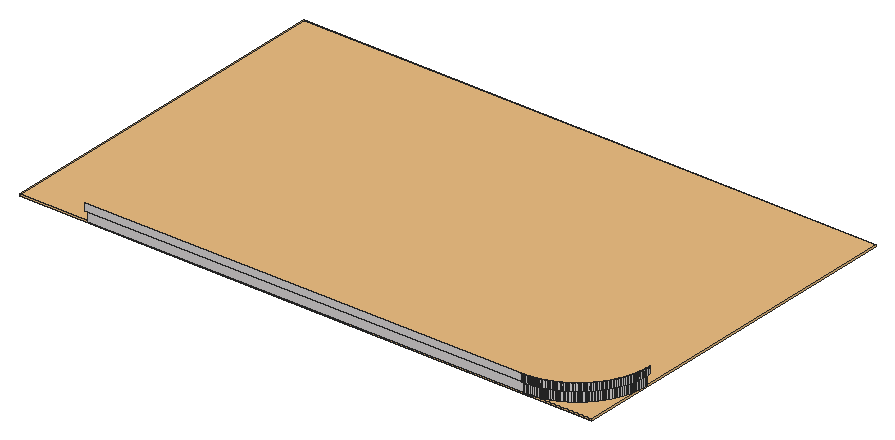
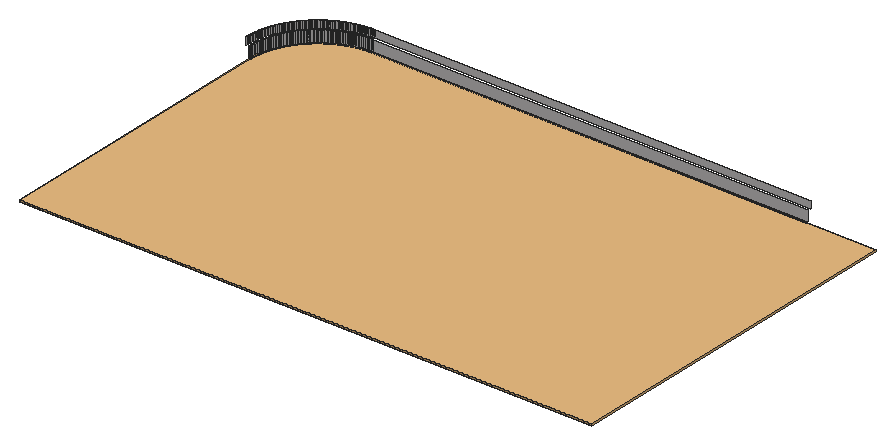
# SketchUp Ruby script. Lengths in inches.
U = 1.inch
M = Sketchup.active_model
def pt(a) = Geom::Point3d.new(a.map { |v| v * U })
def face(e, loops, mat)
  f = e.add_face(loops[0].map { |a| pt(a) })
  loops[1..].each { |l| e.add_face(l.map { |a| pt(a) }).erase! }
  f.material = f.back_material = mat if mat
  f
end
# faces: each face lists its corners as indices into pts; further lists are holes
def faces(e, pts, list, mat = nil) = list.each { |f| face(e, (f[0].is_a?(Array) ? f : [f]).map { |l| l.map { |i| pts[i] } }, mat) }
# xy, xz, yz: faces in a plane at the given z, y or x. An outline is a flat list of corners, or four numbers for a rectangle; further outlines are holes
def ring(l) = l.size == 4 ? [[l[0], l[1]], [l[2], l[1]], [l[2], l[3]], [l[0], l[3]]] : l.each_slice(2).to_a
def flat(e, list, mat, &to3) = list.each { |f| face(e, (f[0].is_a?(Array) ? f : [f]).map { |l| ring(l).map { |u, v| to3.(u, v) } }, mat) }
def xy(e, z, list, mat = nil) = flat(e, list, mat) { |x, y| [x, y, z] }
def xz(e, y, list, mat = nil) = flat(e, list, mat) { |x, z| [x, y, z] }
def yz(e, x, list, mat = nil) = flat(e, list, mat) { |y, z| [x, y, z] }
def lines(e, pts, list) = list.each { |a, b| e.add_line(pt(pts[a]), pt(pts[b])) }
# prism: a flat outline (further loops are holes) pulled along v
def prism(e, loops, v, mat = nil)
  f = face(e, loops, mat); d = Geom::Vector3d.new(v.map { |x| x * U })
  f.pushpull(f.normal.samedirection?(d) ? d.length : -d.length)
end
def box(e, o, s, mat = nil) = prism(e, [[o, [o[0] + s[0], o[1], o[2]], [o[0] + s[0], o[1] + s[1], o[2]], [o[0], o[1] + s[1], o[2]]]], [0, 0, s[2]], mat)
def at(x, y, z, deg = 0) = Geom::Transformation.translation(pt([x, y, z])) * Geom::Transformation.rotation(ORIGIN, Z_AXIS, deg.degrees)
def axes(o, x, y, z) = Geom::Transformation.new([*x, 0, *y, 0, *z, 0, *pt(o).to_a, 1])
def part(name) = M.definitions.add(name)
# library, detail: a bought-in or finely detailed component or shape, given as its bounding box
def library(name, o, s) = part(name).tap { |d| box(d.entities, o, s) }
def detail(e, o, s) = box(e.add_group.entities, o, s)
def put(e, d, t, mat = nil) = e.add_instance(d, t).tap { |i| i.material = mat if mat }
def group(e, t, mat = nil) = e.add_group.tap { |g| g.transformation = t; g.material = mat if mat }.entities
root = M.entities
M.materials.add("Outer Light - 1").color = [251, 216, 141]
M.materials.add("[Quartz Light Brown]").color = [215, 212, 212]
c1 = library("Group\#52",[-0.5,-0.5,0],[314,195,1])
xz(root,281.2,[[225,493,464,497],[464,493,464.52,497]],"[Quartz Light Brown]")
xz(root,282.7,[[225,487,464,493],[464,487,464.5,493]],"[Quartz Light Brown]")
xz(root,283.7,[[225,486,464,487],[464,486,464.48,487]],"[Quartz Light Brown]")
yz(root,501,[[320.22,486,320.7,487]],"[Quartz Light Brown]")
yz(root,502,[[320.2,487,320.7,493]],"[Quartz Light Brown]")
yz(root,503.5,[[320.18,493,320.7,497]],"[Quartz Light Brown]")
p = [[464.48,283.7,486],[464.97,283.71,486],[464.97,283.71,487],[464.48,283.7,487],[465.45,283.73,486],[465.45,283.73,487],
  [465.9375,283.75,486],[465.9375,283.75,487],[466.42,283.78,486],[466.42,283.78,487],[466.9,283.82,486],[466.9,283.82,487],
  [467.39,283.86,486],[467.39,283.86,487],[467.87,283.9,486],[467.87,283.9,487],[468.35,283.96,486],[468.35,283.96,487],
  [468.83,284.02,486],[468.83,284.02,487],[469.31,284.08,486],[469.31,284.08,487],[469.79,284.16,486],[469.79,284.16,487],
  [470.27,284.24,486],[470.27,284.24,487],[470.74,284.32,486],[470.74,284.32,487],[471.22,284.41,486],[471.22,284.41,487],
  [471.69,284.51,486],[471.69,284.51,487],[472.17,284.61,486],[472.17,284.61,487],[472.64,284.72,486],[472.64,284.72,487],
  [473.11,284.84,486],[473.11,284.84,487],[473.58,284.96,486],[473.58,284.96,487],[474.04,285.09,486],[474.04,285.09,487],
  [474.51,285.22,486],[474.51,285.22,487],[474.97,285.37,486],[474.97,285.37,487],[475.43,285.51,486],[475.43,285.51,487],
  [475.89,285.66,486],[475.89,285.66,487],[476.35,285.82,486],[476.35,285.82,487],[476.81,285.99,486],[476.81,285.99,487],
  [477.26,286.16,486],[477.26,286.16,487],[477.71,286.34,486],[477.71,286.34,487],[478.16,286.52,486],[478.16,286.52,487],
  [478.61,286.71,486],[478.61,286.71,487],[479.05,286.9,486],[479.05,286.9,487],[479.49,287.1,486],[479.49,287.1,487],
  [479.93,287.31,486],[479.93,287.31,487],[480.36,287.52,486],[480.36,287.52,487],[480.8,287.73,486],[480.8,287.73,487],
  [481.23,287.96,486],[481.23,287.96,487],[481.65,288.18,486],[481.65,288.18,487],[482.08,288.42,486],[482.08,288.42,487],
  [482.5,288.66,486],[482.5,288.66,487],[482.92,288.9,486],[482.92,288.9,487],[483.33,289.15,486],[483.33,289.15,487],
  [483.74,289.41,486],[483.74,289.41,487],[484.15,289.67,486],[484.15,289.67,487],[484.56,289.9375,486],[484.56,289.9375,487],
  [484.96,290.21,486],[484.96,290.21,487],[485.35,290.49,486],[485.35,290.49,487],[485.75,290.77,486],[485.75,290.77,487],
  [486.14,291.05,486],[486.14,291.05,487],[486.52,291.35,486],[486.52,291.35,487],[486.91,291.64,486],[486.91,291.64,487],
  [487.28,291.95,486],[487.28,291.95,487],[487.66,292.25,486],[487.66,292.25,487],[488.03,292.57,486],[488.03,292.57,487],
  [488.4,292.88,486],[488.4,292.88,487],[488.76,293.2,486],[488.76,293.2,487],[489.12,293.53,486],[489.12,293.53,487],
  [489.47,293.86,486],[489.47,293.86,487],[489.82,294.2,486],[489.82,294.2,487],[490.16,294.54,486],[490.16,294.54,487],
  [490.5,294.88,486],[490.5,294.88,487],[490.84,295.23,486],[490.84,295.23,487],[491.17,295.59,486],[491.17,295.59,487],
  [491.5,295.94,486],[491.5,295.94,487],[491.82,296.31,486],[491.82,296.31,487],[492.14,296.67,486],[492.14,296.67,487],
  [492.45,297.04,486],[492.45,297.04,487],[492.75,297.42,486],[492.75,297.42,487],[493.06,297.79,486],[493.06,297.79,487],
  [493.35,298.18,486],[493.35,298.18,487],[493.65,298.5625,486],[493.65,298.5625,487],[493.93,298.95,486],[493.93,298.95,487],
  [494.22,299.35,486],[494.22,299.35,487],[494.49,299.74,486],[494.49,299.74,487],[494.76,300.14,486],[494.76,300.14,487],
  [495.03,300.55,486],[495.03,300.55,487],[495.29,300.96,486],[495.29,300.96,487],[495.55,301.37,486],[495.55,301.37,487],
  [495.8,301.78,486],[495.8,301.78,487],[496.04,302.2,486],[496.04,302.2,487],[496.28,302.62,486],[496.28,302.62,487],
  [496.52,303.05,486],[496.52,303.05,487],[496.74,303.47,486],[496.74,303.47,487],[496.97,303.9,486],[496.97,303.9,487],
  [497.18,304.34,486],[497.18,304.34,487],[497.4,304.77,486],[497.4,304.77,487],[497.6,305.21,486],[497.6,305.21,487],
  [497.8,305.65,486],[497.8,305.65,487],[498,306.1,486],[498,306.1,487],[498.18,306.54,486],[498.18,306.54,487],
  [498.37,306.99,486],[498.37,306.99,487],[498.54,307.44,486],[498.54,307.44,487],[498.71,307.89,486],[498.71,307.89,487],
  [498.88,308.35,486],[498.88,308.35,487],[499.04,308.81,486],[499.04,308.81,487],[499.1875,309.27,486],[499.1875,309.27,487],
  [499.34,309.73,486],[499.34,309.73,487],[499.48,310.19,486],[499.48,310.19,487],[499.61,310.66,486],[499.61,310.66,487],
  [499.74,311.125,486],[499.74,311.125,487],[499.86,311.59,486],[499.86,311.59,487],[499.98,312.0625,486],[499.98,312.0625,487],
  [500.09,312.54,486],[500.09,312.54,487],[500.19,313.01,486],[500.19,313.01,487],[500.29,313.48,486],[500.29,313.48,487],
  [500.38,313.96,486],[500.38,313.96,487],[500.47,314.44,486],[500.47,314.44,487],[500.54,314.91,486],[500.54,314.91,487],
  [500.62,315.39,486],[500.62,315.39,487],[500.68,315.87,486],[500.68,315.87,487],[500.74,316.35,486],[500.74,316.35,487],
  [500.8,316.83,486],[500.8,316.83,487],[500.84,317.32,486],[500.84,317.32,487],[500.89,317.8,486],[500.89,317.8,487],
  [500.92,318.28,486],[500.92,318.28,487],[500.95,318.76,486],[500.95,318.76,487],[500.97,319.25,486],[500.97,319.25,487],
  [500.99,319.73,486],[500.99,319.73,487],[501,320.22,486],[501,320.22,487],[464.99,282.71,487],[464.99,282.71,493],
  [464.5,282.7,493],[464.5,282.7,487],[465.49,282.73,487],[465.49,282.73,493],[465.99,282.75,487],[465.99,282.75,493],
  [466.49,282.78,487],[466.49,282.78,493],[466.98,282.82,487],[466.98,282.82,493],[467.48,282.86,487],[467.48,282.86,493],
  [467.97,282.91,487],[467.97,282.91,493],[468.47,282.96,487],[468.47,282.96,493],[468.96,283.03,487],[468.96,283.03,493],
  [469.45,283.09,487],[469.45,283.09,493],[469.94,283.17,487],[469.94,283.17,493],[470.44,283.25,487],[470.44,283.25,493],
  [470.92,283.34,487],[470.92,283.34,493],[471.41,283.43,487],[471.41,283.43,493],[471.9,283.53,487],[471.9,283.53,493],
  [472.39,283.64,487],[472.39,283.64,493],[472.87,283.75,487],[472.87,283.75,493],[473.35,283.87,487],[473.35,283.87,493],
  [473.84,284,487],[473.84,284,493],[474.31,284.13,487],[474.31,284.13,493],[474.79,284.27,487],[474.79,284.27,493],
  [475.27,284.41,487],[475.27,284.41,493],[475.74,284.5625,487],[475.74,284.5625,493],[476.21,284.72,487],[476.21,284.72,493],
  [476.68,284.88,487],[476.68,284.88,493],[477.15,285.05,487],[477.15,285.05,493],[477.62,285.22,487],[477.62,285.22,493],
  [478.08,285.41,487],[478.08,285.41,493],[478.54,285.59,487],[478.54,285.59,493],[479,285.79,487],[479,285.79,493],
  [479.46,285.99,487],[479.46,285.99,493],[479.91,286.19,487],[479.91,286.19,493],[480.36,286.4,487],[480.36,286.4,493],
  [480.81,286.62,487],[480.81,286.62,493],[481.25,286.84,487],[481.25,286.84,493],[481.69,287.07,487],[481.69,287.07,493],
  [482.13,287.31,487],[482.13,287.31,493],[482.57,287.55,487],[482.57,287.55,493],[483,287.79,487],[483,287.79,493],
  [483.43,288.04,487],[483.43,288.04,493],[483.85,288.3,487],[483.85,288.3,493],[484.28,288.5625,487],[484.28,288.5625,493],
  [484.7,288.83,487],[484.7,288.83,493],[485.11,289.11,487],[485.11,289.11,493],[485.52,289.38,487],[485.52,289.38,493],
  [485.93,289.67,487],[485.93,289.67,493],[486.34,289.96,487],[486.34,289.96,493],[486.74,290.25,487],[486.74,290.25,493],
  [487.13,290.55,487],[487.13,290.55,493],[487.53,290.86,487],[487.53,290.86,493],[487.91,291.17,487],[487.91,291.17,493],
  [488.3,291.49,487],[488.3,291.49,493],[488.68,291.81,487],[488.68,291.81,493],[489.06,292.13,487],[489.06,292.13,493],
  [489.43,292.46,487],[489.43,292.46,493],[489.79,292.8,487],[489.79,292.8,493],[490.16,293.14,487],[490.16,293.14,493],
  [490.52,293.48,487],[490.52,293.48,493],[490.87,293.83,487],[490.87,293.83,493],[491.22,294.18,487],[491.22,294.18,493],
  [491.5625,294.54,487],[491.5625,294.54,493],[491.9,294.91,487],[491.9,294.91,493],[492.24,295.27,487],[492.24,295.27,493],
  [492.57,295.65,487],[492.57,295.65,493],[492.9,296.02,487],[492.9,296.02,493],[493.22,296.4,487],[493.22,296.4,493],
  [493.53,296.79,487],[493.53,296.79,493],[493.84,297.18,487],[493.84,297.18,493],[494.15,297.57,487],[494.15,297.57,493],
  [494.45,297.96,487],[494.45,297.96,493],[494.74,298.37,487],[494.74,298.37,493],[495.03,298.77,487],[495.03,298.77,493],
  [495.32,299.18,487],[495.32,299.18,493],[495.6,299.59,487],[495.6,299.59,493],[495.87,300,487],[495.87,300,493],
  [496.14,300.42,487],[496.14,300.42,493],[496.4,300.85,487],[496.4,300.85,493],[496.66,301.27,487],[496.66,301.27,493],
  [496.91,301.7,487],[496.91,301.7,493],[497.15,302.13,487],[497.15,302.13,493],[497.4,302.57,487],[497.4,302.57,493],
  [497.63,303.01,487],[497.63,303.01,493],[497.86,303.45,487],[497.86,303.45,493],[498.08,303.89,487],[498.08,303.89,493],
  [498.3,304.34,487],[498.3,304.34,493],[498.51,304.79,487],[498.51,304.79,493],[498.71,305.25,487],[498.71,305.25,493],
  [498.91,305.7,487],[498.91,305.7,493],[499.11,306.16,487],[499.11,306.16,493],[499.29,306.62,487],[499.29,306.62,493],
  [499.48,307.08,487],[499.48,307.08,493],[499.65,307.55,487],[499.65,307.55,493],[499.82,308.02,487],[499.82,308.02,493],
  [499.98,308.49,487],[499.98,308.49,493],[500.14,308.96,487],[500.14,308.96,493],[500.29,309.43,487],[500.29,309.43,493],
  [500.44,309.91,487],[500.44,309.91,493],[500.57,310.39,487],[500.57,310.39,493],[500.71,310.87,487],[500.71,310.87,493],
  [500.83,311.35,487],[500.83,311.35,493],[500.95,311.83,487],[500.95,311.83,493],[501.0625,312.31,487],[501.0625,312.31,493],
  [501.17,312.8,487],[501.17,312.8,493],[501.27,313.29,487],[501.27,313.29,493],[501.36,313.78,487],[501.36,313.78,493],
  [501.45,314.27,487],[501.45,314.27,493],[501.53,314.76,487],[501.53,314.76,493],[501.61,315.25,487],[501.61,315.25,493],
  [501.67,315.74,487],[501.67,315.74,493],[501.74,316.23,487],[501.74,316.23,493],[501.79,316.73,487],[501.79,316.73,493],
  [501.84,317.22,487],[501.84,317.22,493],[501.88,317.72,487],[501.88,317.72,493],[501.92,318.22,487],[501.92,318.22,493],
  [501.95,318.71,487],[501.95,318.71,493],[501.97,319.21,487],[501.97,319.21,493],[501.99,319.71,487],[501.99,319.71,493],
  [502,320.2,487],[502,320.2,493],[464.52,281.2,493],[465.03,281.21,493],[465.03,281.21,497],[464.52,281.2,497],
  [465.55,281.23,493],[465.55,281.23,497],[466.07,281.26,493],[466.07,281.26,497],[466.58,281.29,493],[466.58,281.29,497],
  [467.1,281.32,493],[467.1,281.32,497],[467.61,281.37,493],[467.61,281.37,497],[468.13,281.42,493],[468.13,281.42,497],
  [468.64,281.47,493],[468.64,281.47,497],[469.16,281.54,493],[469.16,281.54,497],[469.67,281.61,493],[469.67,281.61,497],
  [470.18,281.6875,493],[470.18,281.6875,497],[470.6875,281.77,493],[470.6875,281.77,497],[471.2,281.86,493],[471.2,281.86,497],
  [471.71,281.96,493],[471.71,281.96,497],[472.21,282.0625,493],[472.21,282.0625,497],[472.72,282.17,493],[472.72,282.17,497],
  [473.22,282.29,493],[473.22,282.29,497],[473.72,282.42,493],[473.72,282.42,497],[474.22,282.55,493],[474.22,282.55,497],
  [474.72,282.68,493],[474.72,282.68,497],[475.22,282.83,493],[475.22,282.83,497],[475.71,282.98,493],[475.71,282.98,497],
  [476.21,283.13,493],[476.21,283.13,497],[476.7,283.3,493],[476.7,283.3,497],[477.19,283.47,493],[477.19,283.47,497],
  [477.67,283.64,493],[477.67,283.64,497],[478.16,283.82,493],[478.16,283.82,497],[478.64,284.01,493],[478.64,284.01,497],
  [479.12,284.21,493],[479.12,284.21,497],[479.59,284.41,493],[479.59,284.41,497],[480.07,284.62,493],[480.07,284.62,497],
  [480.54,284.83,493],[480.54,284.83,497],[481.01,285.05,493],[481.01,285.05,497],[481.47,285.27,493],[481.47,285.27,497],
  [481.93,285.51,493],[481.93,285.51,497],[482.39,285.74,493],[482.39,285.74,497],[482.85,285.99,493],[482.85,285.99,497],
  [483.3,286.24,493],[483.3,286.24,497],[483.75,286.49,493],[483.75,286.49,497],[484.2,286.75,493],[484.2,286.75,497],
  [484.64,287.02,493],[484.64,287.02,497],[485.08,287.29,493],[485.08,287.29,497],[485.51,287.57,493],[485.51,287.57,497],
  [485.95,287.86,493],[485.95,287.86,497],[486.375,288.15,493],[486.375,288.15,497],[486.8,288.44,493],[486.8,288.44,497],
  [487.22,288.74,493],[487.22,288.74,497],[487.63,289.05,493],[487.63,289.05,497],[488.05,289.36,493],[488.05,289.36,497],
  [488.45,289.68,493],[488.45,289.68,497],[488.86,290,493],[488.86,290,497],[489.26,290.33,493],[489.26,290.33,497],
  [489.65,290.66,493],[489.65,290.66,497],[490.04,291,493],[490.04,291,497],[490.43,291.35,493],[490.43,291.35,497],
  [490.8125,291.7,493],[490.8125,291.7,497],[491.19,292.05,493],[491.19,292.05,497],[491.5625,292.41,493],[491.5625,292.41,497],
  [491.93,292.77,493],[491.93,292.77,497],[492.29,293.14,493],[492.29,293.14,497],[492.65,293.51,493],[492.65,293.51,497],
  [493.01,293.89,493],[493.01,293.89,497],[493.35,294.27,493],[493.35,294.27,497],[493.7,294.66,493],[493.7,294.66,497],
  [494.04,295.05,493],[494.04,295.05,497],[494.37,295.44,493],[494.37,295.44,497],[494.7,295.84,493],[494.7,295.84,497],
  [495.02,296.25,493],[495.02,296.25,497],[495.34,296.65,493],[495.34,296.65,497],[495.65,297.07,493],[495.65,297.07,497],
  [495.96,297.48,493],[495.96,297.48,497],[496.26,297.9,493],[496.26,297.9,497],[496.55,298.33,493],[496.55,298.33,497],
  [496.84,298.76,493],[496.84,298.76,497],[497.13,299.1875,493],[497.13,299.1875,497],[497.41,299.625,493],[497.41,299.625,497],
  [497.68,300.0625,493],[497.68,300.0625,497],[497.95,300.5,493],[497.95,300.5,497],[498.21,300.95,493],[498.21,300.95,497],
  [498.46,301.4,493],[498.46,301.4,497],[498.71,301.85,493],[498.71,301.85,497],[498.96,302.31,493],[498.96,302.31,497],
  [499.19,302.77,493],[499.19,302.77,497],[499.43,303.23,493],[499.43,303.23,497],[499.65,303.7,493],[499.65,303.7,497],
  [499.87,304.16,493],[499.87,304.16,497],[500.09,304.63,493],[500.09,304.63,497],[500.29,305.11,493],[500.29,305.11,497],
  [500.49,305.59,493],[500.49,305.59,497],[500.6875,306.0625,493],[500.6875,306.0625,497],[500.875,306.55,493],[500.875,306.55,497],
  [501.06,307.03,493],[501.06,307.03,497],[501.23,307.52,493],[501.23,307.52,497],[501.4,308,493],[501.4,308,497],
  [501.57,308.49,493],[501.57,308.49,497],[501.72,308.99,493],[501.72,308.99,497],[501.875,309.48,493],[501.875,309.48,497],
  [502.02,309.98,493],[502.02,309.98,497],[502.15,310.48,493],[502.15,310.48,497],[502.28,310.98,493],[502.28,310.98,497],
  [502.41,311.48,493],[502.41,311.48,497],[502.53,311.98,493],[502.53,311.98,497],[502.64,312.49,493],[502.64,312.49,497],
  [502.74,312.99,493],[502.74,312.99,497],[502.84,313.5,493],[502.84,313.5,497],[502.93,314.01,493],[502.93,314.01,497],
  [503.01,314.52,493],[503.01,314.52,497],[503.09,315.03,493],[503.09,315.03,497],[503.16,315.55,493],[503.16,315.55,497],
  [503.23,316.06,493],[503.23,316.06,497],[503.28,316.57,493],[503.28,316.57,497],[503.33,317.09,493],[503.33,317.09,497],
  [503.38,317.6,493],[503.38,317.6,497],[503.42,318.12,493],[503.42,318.12,497],[503.45,318.63,493],[503.45,318.63,497],
  [503.47,319.15,493],[503.47,319.15,497],[503.49,319.67,493],[503.49,319.67,497],[503.5,320.18,493],[503.5,320.18,497],
  [464,283.7,487],[464,283.7,493],[502,320.7,493],[502,320.7,495]]
faces(root,p,[[0,1,2,3],[1,4,5,2],[4,6,7,5],[6,8,9,7],[8,10,11,9],[10,12,13,11],[12,14,15,13],[14,16,17,15],
  [16,18,19,17],[18,20,21,19],[20,22,23,21],[22,24,25,23],[24,26,27,25],[26,28,29,27],[28,30,31,29],[30,32,33,31],
  [32,34,35,33],[34,36,37,35],[36,38,39,37],[38,40,41,39],[40,42,43,41],[42,44,45,43],[44,46,47,45],[46,48,49,47],
  [48,50,51,49],[50,52,53,51],[52,54,55,53],[54,56,57,55],[56,58,59,57],[58,60,61,59],[60,62,63,61],[62,64,65,63],
  [64,66,67,65],[66,68,69,67],[68,70,71,69],[70,72,73,71],[72,74,75,73],[74,76,77,75],[76,78,79,77],[78,80,81,79],
  [80,82,83,81],[82,84,85,83],[84,86,87,85],[86,88,89,87],[88,90,91,89],[90,92,93,91],[92,94,95,93],[94,96,97,95],
  [96,98,99,97],[98,100,101,99],[100,102,103,101],[102,104,105,103],[104,106,107,105],[106,108,109,107],[108,110,111,109],[110,112,113,111],
  [112,114,115,113],[114,116,117,115],[116,118,119,117],[118,120,121,119],[120,122,123,121],[122,124,125,123],[124,126,127,125],[126,128,129,127],
  [128,130,131,129],[130,132,133,131],[132,134,135,133],[134,136,137,135],[136,138,139,137],[138,140,141,139],[140,142,143,141],[142,144,145,143],
  [144,146,147,145],[146,148,149,147],[148,150,151,149],[150,152,153,151],[152,154,155,153],[154,156,157,155],[156,158,159,157],[158,160,161,159],
  [160,162,163,161],[162,164,165,163],[164,166,167,165],[166,168,169,167],[168,170,171,169],[170,172,173,171],[172,174,175,173],[174,176,177,175],
  [176,178,179,177],[178,180,181,179],[180,182,183,181],[182,184,185,183],[184,186,187,185],[186,188,189,187],[188,190,191,189],[190,192,193,191],
  [192,194,195,193],[194,196,197,195],[196,198,199,197],[198,200,201,199],[200,202,203,201],[202,204,205,203],[204,206,207,205],[206,208,209,207],
  [208,210,211,209],[210,212,213,211],[212,214,215,213],[214,216,217,215],[216,218,219,217],[218,220,221,219],[220,222,223,221],[222,224,225,223],
  [224,226,227,225],[226,228,229,227],[228,230,231,229],[230,232,233,231],[232,234,235,233],[234,236,237,235],[238,239,240,241],[242,243,239,238],
  [244,245,243,242],[246,247,245,244],[248,249,247,246],[250,251,249,248],[252,253,251,250],[254,255,253,252],[256,257,255,254],[258,259,257,256],
  [260,261,259,258],[262,263,261,260],[264,265,263,262],[266,267,265,264],[268,269,267,266],[270,271,269,268],[272,273,271,270],[274,275,273,272],
  [276,277,275,274],[278,279,277,276],[280,281,279,278],[282,283,281,280],[284,285,283,282],[286,287,285,284],[288,289,287,286],[290,291,289,288],
  [292,293,291,290],[294,295,293,292],[296,297,295,294],[298,299,297,296],[300,301,299,298],[302,303,301,300],[304,305,303,302],[306,307,305,304],
  [308,309,307,306],[310,311,309,308],[312,313,311,310],[314,315,313,312],[316,317,315,314],[318,319,317,316],[320,321,319,318],[322,323,321,320],
  [324,325,323,322],[326,327,325,324],[328,329,327,326],[330,331,329,328],[332,333,331,330],[334,335,333,332],[336,337,335,334],[338,339,337,336],
  [340,341,339,338],[342,343,341,340],[344,345,343,342],[346,347,345,344],[348,349,347,346],[350,351,349,348],[352,353,351,350],[354,355,353,352],
  [356,357,355,354],[358,359,357,356],[360,361,359,358],[362,363,361,360],[364,365,363,362],[366,367,365,364],[368,369,367,366],[370,371,369,368],
  [372,373,371,370],[374,375,373,372],[376,377,375,374],[378,379,377,376],[380,381,379,378],[382,383,381,380],[384,385,383,382],[386,387,385,384],
  [388,389,387,386],[390,391,389,388],[392,393,391,390],[394,395,393,392],[396,397,395,394],[398,399,397,396],[400,401,399,398],[402,403,401,400],
  [404,405,403,402],[406,407,405,404],[408,409,407,406],[410,411,409,408],[412,413,411,410],[414,415,413,412],[416,417,415,414],[418,419,417,416],
  [420,421,419,418],[422,423,421,420],[424,425,423,422],[426,427,425,424],[428,429,427,426],[430,431,429,428],[432,433,431,430],[434,435,433,432],
  [436,437,435,434],[438,439,437,436],[440,441,439,438],[442,443,441,440],[444,445,443,442],[446,447,445,444],[448,449,447,446],[450,451,449,448],
  [452,453,451,450],[454,455,453,452],[456,457,455,454],[458,459,457,456],[460,461,459,458],[462,463,461,460],[464,465,463,462],[466,467,465,464],
  [468,469,467,466],[470,471,469,468],[472,473,471,470],[474,475,473,472],[476,477,478,479],[477,480,481,478],[480,482,483,481],[482,484,485,483],
  [484,486,487,485],[486,488,489,487],[488,490,491,489],[490,492,493,491],[492,494,495,493],[494,496,497,495],[496,498,499,497],[498,500,501,499],
  [500,502,503,501],[502,504,505,503],[504,506,507,505],[506,508,509,507],[508,510,511,509],[510,512,513,511],[512,514,515,513],[514,516,517,515],
  [516,518,519,517],[518,520,521,519],[520,522,523,521],[522,524,525,523],[524,526,527,525],[526,528,529,527],[528,530,531,529],[530,532,533,531],
  [532,534,535,533],[534,536,537,535],[536,538,539,537],[538,540,541,539],[540,542,543,541],[542,544,545,543],[544,546,547,545],[546,548,549,547],
  [548,550,551,549],[550,552,553,551],[552,554,555,553],[554,556,557,555],[556,558,559,557],[558,560,561,559],[560,562,563,561],[562,564,565,563],
  [564,566,567,565],[566,568,569,567],[568,570,571,569],[570,572,573,571],[572,574,575,573],[574,576,577,575],[576,578,579,577],[578,580,581,579],
  [580,582,583,581],[582,584,585,583],[584,586,587,585],[586,588,589,587],[588,590,591,589],[590,592,593,591],[592,594,595,593],[594,596,597,595],
  [596,598,599,597],[598,600,601,599],[600,602,603,601],[602,604,605,603],[604,606,607,605],[606,608,609,607],[608,610,611,609],[610,612,613,611],
  [612,614,615,613],[614,616,617,615],[616,618,619,617],[618,620,621,619],[620,622,623,621],[622,624,625,623],[624,626,627,625],[626,628,629,627],
  [628,630,631,629],[630,632,633,631],[632,634,635,633],[634,636,637,635],[636,638,639,637],[638,640,641,639],[640,642,643,641],[642,644,645,643],
  [644,646,647,645],[646,648,649,647],[648,650,651,649],[650,652,653,651],[652,654,655,653],[654,656,657,655],[656,658,659,657],[658,660,661,659],
  [660,662,663,661],[662,664,665,663],[664,666,667,665],[666,668,669,667],[668,670,671,669],[670,672,673,671],[672,674,675,673],[674,676,677,675],
  [676,678,679,677],[678,680,681,679],[680,682,683,681],[682,684,685,683],[684,686,687,685],[686,688,689,687],[688,690,691,689],[690,692,693,691],
  [692,694,695,693],[694,696,697,695],[696,698,699,697],[698,700,701,699],[700,702,703,701],[702,704,705,703],[704,706,707,705],[706,708,709,707],
  [708,710,711,709],[710,712,713,711]],"[Quartz Light Brown]")
lines(root,p,[[714,715],[716,717]])
put(root,c1,at(188,283.7,486),"Outer Light - 1")
